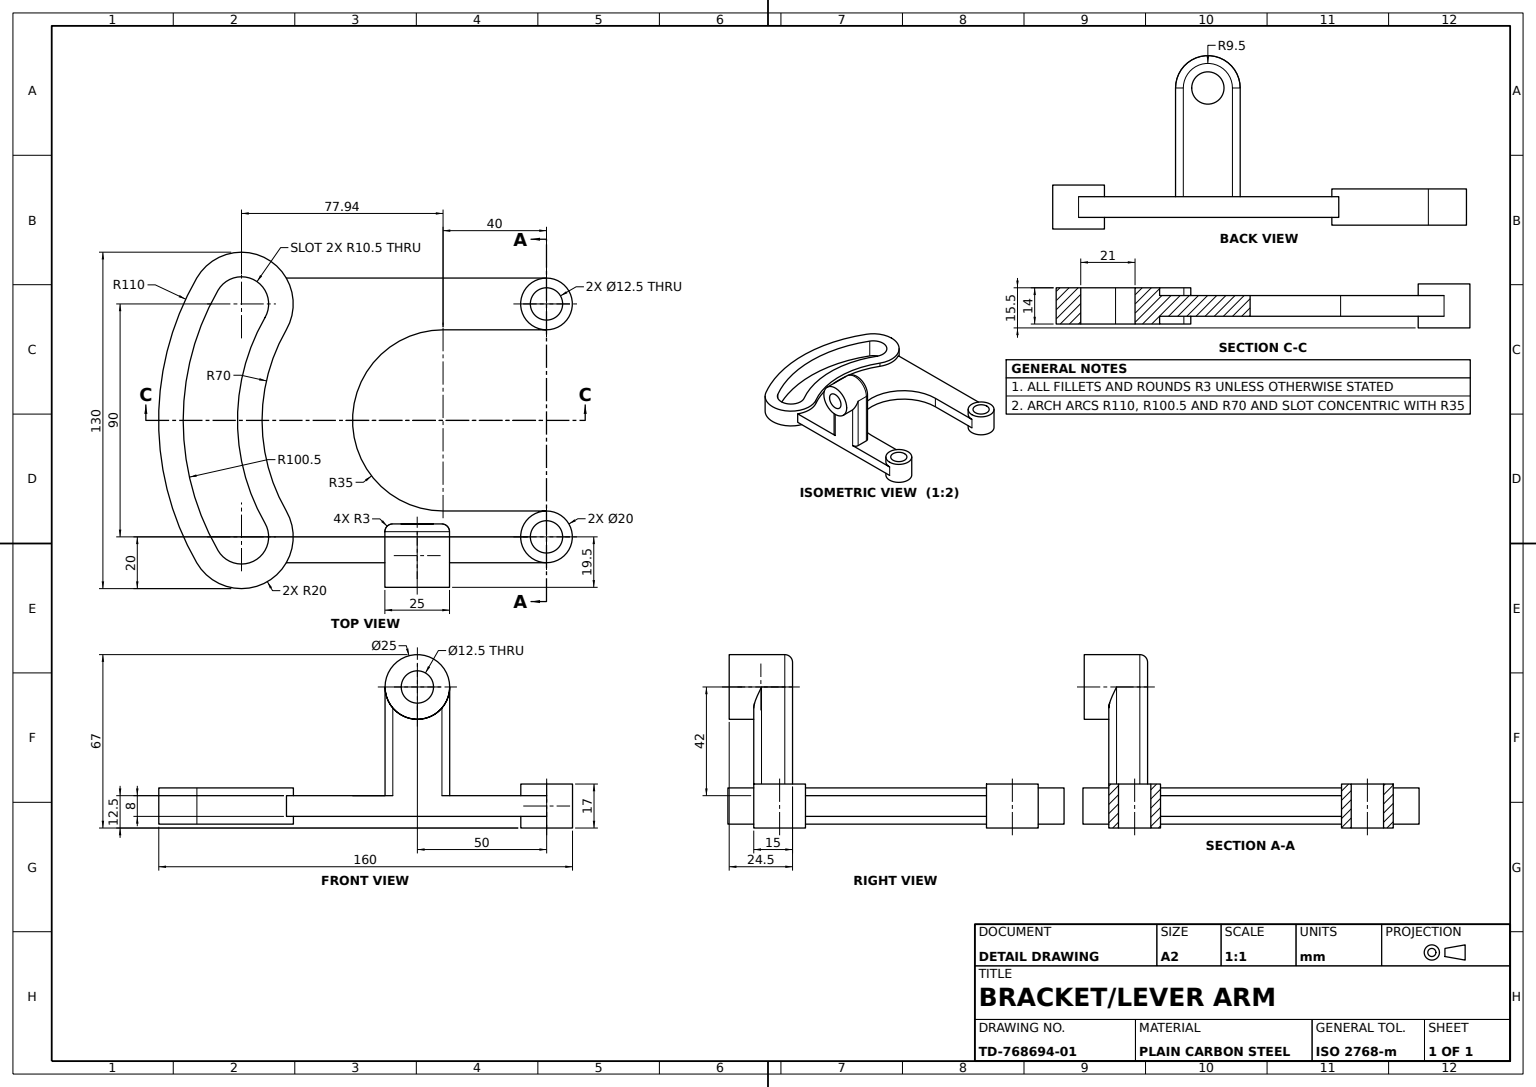
ISO-10303-21;
HEADER;
FILE_DESCRIPTION((''),'2;1');
FILE_NAME('','',(''),(''),'','','');
FILE_SCHEMA(('AUTOMOTIVE_DESIGN'));
ENDSEC;
DATA;
#1=APPLICATION_CONTEXT('');
#2=PRODUCT_CONTEXT('',#1,'mechanical');
#3=PRODUCT('','','',(#2));
#4=PRODUCT_DEFINITION_FORMATION('','',#3);
#5=PRODUCT_DEFINITION_CONTEXT('',#1,'design');
#6=PRODUCT_DEFINITION('','',#4,#5);
#7=PRODUCT_DEFINITION_SHAPE('','',#6);
#8=(LENGTH_UNIT()NAMED_UNIT(*)SI_UNIT(.MILLI.,.METRE.));
#9=(NAMED_UNIT(*)PLANE_ANGLE_UNIT()SI_UNIT($,.RADIAN.));
#10=(NAMED_UNIT(*)SI_UNIT($,.STERADIAN.)SOLID_ANGLE_UNIT());
#11=UNCERTAINTY_MEASURE_WITH_UNIT(LENGTH_MEASURE(1.E-05),#8,'distance_accuracy_value','');
#12=(GEOMETRIC_REPRESENTATION_CONTEXT(3)GLOBAL_UNCERTAINTY_ASSIGNED_CONTEXT((#11))GLOBAL_UNIT_ASSIGNED_CONTEXT((#8,#9,#10))REPRESENTATION_CONTEXT('',''));
#13=CARTESIAN_POINT('',(0.,-4.,-80.));
#14=VERTEX_POINT('',#13);
#15=CARTESIAN_POINT('',(0.,-8.5,-80.));
#16=VERTEX_POINT('',#15);
#17=CARTESIAN_POINT('',(0.,8.5,-80.));
#18=DIRECTION('',(0.,-1.,0.));
#19=VECTOR('',#18,1000.);
#20=LINE('',#17,#19);
#21=EDGE_CURVE('',#14,#16,#20,.T.);
#22=ORIENTED_EDGE('',*,*,#21,.T.);
#23=CARTESIAN_POINT('',(0.,-8.5,-100.));
#24=VERTEX_POINT('',#23);
#25=CARTESIAN_POINT('',(0.,-8.5,-90.));
#26=DIRECTION('',(0.,1.,0.));
#27=DIRECTION('',(0.,0.,1.));
#28=AXIS2_PLACEMENT_3D('',#25,#26,#27);
#29=CIRCLE('',#28,10.);
#30=EDGE_CURVE('',#16,#24,#29,.T.);
#31=ORIENTED_EDGE('',*,*,#30,.T.);
#32=CARTESIAN_POINT('',(0.,-4.,-100.));
#33=VERTEX_POINT('',#32);
#34=CARTESIAN_POINT('',(0.,8.5,-100.));
#35=LINE('',#34,#19);
#36=EDGE_CURVE('',#33,#24,#35,.T.);
#37=ORIENTED_EDGE('',*,*,#36,.F.);
#38=CARTESIAN_POINT('',(0.,4.,-100.));
#39=VERTEX_POINT('',#38);
#40=LINE('',#38,#19);
#41=EDGE_CURVE('',#39,#33,#40,.T.);
#42=ORIENTED_EDGE('',*,*,#41,.F.);
#43=VERTEX_POINT('',#34);
#44=EDGE_CURVE('',#43,#39,#35,.T.);
#45=ORIENTED_EDGE('',*,*,#44,.F.);
#46=VERTEX_POINT('',#17);
#47=CARTESIAN_POINT('',(0.,8.5,-90.));
#48=AXIS2_PLACEMENT_3D('',#47,#26,#27);
#49=CIRCLE('',#48,10.);
#50=EDGE_CURVE('',#46,#43,#49,.T.);
#51=ORIENTED_EDGE('',*,*,#50,.F.);
#52=CARTESIAN_POINT('',(0.,4.,-80.));
#53=VERTEX_POINT('',#52);
#54=EDGE_CURVE('',#46,#53,#20,.T.);
#55=ORIENTED_EDGE('',*,*,#54,.T.);
#56=LINE('',#52,#19);
#57=EDGE_CURVE('',#53,#14,#56,.T.);
#58=ORIENTED_EDGE('',*,*,#57,.T.);
#59=EDGE_LOOP('',(#22,#31,#37,#42,#45,#51,#55,#58));
#60=FACE_OUTER_BOUND('',#59,.T.);
#61=DIRECTION('',(0.,0.,-1.));
#62=AXIS2_PLACEMENT_3D('',#47,#18,#61);
#63=CYLINDRICAL_SURFACE('',#62,10.);
#64=ADVANCED_FACE('',(#60),#63,.T.);
#65=CARTESIAN_POINT('',(-117.942286,-7.,-110.));
#66=VERTEX_POINT('',#65);
#67=CARTESIAN_POINT('',(-135.262794,-7.,-100.));
#68=VERTEX_POINT('',#67);
#69=CARTESIAN_POINT('',(-117.942286,-7.,-90.));
#70=AXIS2_PLACEMENT_3D('',#69,#26,#27);
#71=CIRCLE('',#70,20.);
#72=EDGE_CURVE('',#66,#68,#71,.T.);
#73=ORIENTED_EDGE('',*,*,#72,.T.);
#74=CARTESIAN_POINT('',(-135.262794,7.,-100.));
#75=VERTEX_POINT('',#74);
#76=LINE('',#74,#19);
#77=EDGE_CURVE('',#75,#68,#76,.T.);
#78=ORIENTED_EDGE('',*,*,#77,.F.);
#79=CARTESIAN_POINT('',(-117.942286,7.,-110.));
#80=VERTEX_POINT('',#79);
#81=CARTESIAN_POINT('',(-117.942286,7.,-90.));
#82=AXIS2_PLACEMENT_3D('',#81,#26,#27);
#83=CIRCLE('',#82,20.);
#84=EDGE_CURVE('',#80,#75,#83,.T.);
#85=ORIENTED_EDGE('',*,*,#84,.F.);
#86=LINE('',#79,#19);
#87=EDGE_CURVE('',#80,#66,#86,.T.);
#88=ORIENTED_EDGE('',*,*,#87,.T.);
#89=EDGE_LOOP('',(#73,#78,#85,#88));
#90=FACE_OUTER_BOUND('',#89,.T.);
#91=AXIS2_PLACEMENT_3D('',#81,#18,#61);
#92=CYLINDRICAL_SURFACE('',#91,20.);
#93=ADVANCED_FACE('',(#90),#92,.T.);
#94=CARTESIAN_POINT('',(0.,-8.5,-96.25));
#95=VERTEX_POINT('',#94);
#96=CARTESIAN_POINT('',(0.,-8.5,-83.75));
#97=VERTEX_POINT('',#96);
#98=CIRCLE('',#28,6.25);
#99=EDGE_CURVE('',#95,#97,#98,.T.);
#100=ORIENTED_EDGE('',*,*,#99,.T.);
#101=EDGE_CURVE('',#97,#95,#98,.T.);
#102=ORIENTED_EDGE('',*,*,#101,.T.);
#103=EDGE_LOOP('',(#100,#102));
#104=FACE_BOUND('',#103,.T.);
#105=ORIENTED_EDGE('',*,*,#30,.F.);
#106=EDGE_CURVE('',#24,#16,#29,.T.);
#107=ORIENTED_EDGE('',*,*,#106,.F.);
#108=EDGE_LOOP('',(#105,#107));
#109=FACE_OUTER_BOUND('',#108,.T.);
#110=PLANE('',#28);
#111=ADVANCED_FACE('',(#104,#109),#110,.F.);
#112=CARTESIAN_POINT('',(-37.5,46.,19.5));
#113=VERTEX_POINT('',#112);
#114=CARTESIAN_POINT('',(-62.5,46.,19.5));
#115=VERTEX_POINT('',#114);
#116=CARTESIAN_POINT('',(-50.,46.,19.5));
#117=DIRECTION('',(1.,0.,0.));
#118=AXIS2_PLACEMENT_3D('',#116,#27,#117);
#119=CIRCLE('',#118,12.5);
#120=EDGE_CURVE('',#113,#115,#119,.T.);
#121=ORIENTED_EDGE('',*,*,#120,.T.);
#122=EDGE_CURVE('',#115,#113,#119,.T.);
#123=ORIENTED_EDGE('',*,*,#122,.T.);
#124=EDGE_LOOP('',(#121,#123));
#125=FACE_OUTER_BOUND('',#124,.T.);
#126=CARTESIAN_POINT('',(-56.25,46.,19.5));
#127=VERTEX_POINT('',#126);
#128=CARTESIAN_POINT('',(-43.75,46.,19.5));
#129=VERTEX_POINT('',#128);
#130=CIRCLE('',#118,6.25);
#131=EDGE_CURVE('',#127,#129,#130,.T.);
#132=ORIENTED_EDGE('',*,*,#131,.F.);
#133=EDGE_CURVE('',#129,#127,#130,.T.);
#134=ORIENTED_EDGE('',*,*,#133,.F.);
#135=EDGE_LOOP('',(#132,#134));
#136=FACE_BOUND('',#135,.T.);
#137=PLANE('',#118);
#138=ADVANCED_FACE('',(#125,#136),#137,.T.);
#139=CARTESIAN_POINT('',(-59.5,46.,-5.));
#140=VERTEX_POINT('',#139);
#141=CARTESIAN_POINT('',(-40.5,46.,-5.));
#142=VERTEX_POINT('',#141);
#143=CARTESIAN_POINT('',(-50.,46.,-5.));
#144=AXIS2_PLACEMENT_3D('',#143,#61,#117);
#145=CIRCLE('',#144,9.5);
#146=EDGE_CURVE('',#140,#142,#145,.T.);
#147=ORIENTED_EDGE('',*,*,#146,.F.);
#148=CARTESIAN_POINT('',(-62.5,46.,-2.));
#149=VERTEX_POINT('',#148);
#150=CARTESIAN_POINT('',(-59.5,46.,-2.));
#151=AXIS2_PLACEMENT_3D('',#150,#26,#27);
#152=CIRCLE('',#151,3.);
#153=EDGE_CURVE('',#140,#149,#152,.T.);
#154=ORIENTED_EDGE('',*,*,#153,.T.);
#155=CARTESIAN_POINT('',(-37.5,46.,-2.));
#156=VERTEX_POINT('',#155);
#157=CARTESIAN_POINT('',(-50.,46.,-2.));
#158=AXIS2_PLACEMENT_3D('',#157,#27,#117);
#159=CIRCLE('',#158,12.5);
#160=EDGE_CURVE('',#156,#149,#159,.T.);
#161=ORIENTED_EDGE('',*,*,#160,.F.);
#162=CARTESIAN_POINT('',(-40.5,46.,-2.));
#163=AXIS2_PLACEMENT_3D('',#162,#26,#27);
#164=CIRCLE('',#163,3.);
#165=EDGE_CURVE('',#156,#142,#164,.T.);
#166=ORIENTED_EDGE('',*,*,#165,.T.);
#167=EDGE_LOOP('',(#147,#154,#161,#166));
#168=FACE_OUTER_BOUND('',#167,.T.);
#169=TOROIDAL_SURFACE('',#158,9.5,3.);
#170=ADVANCED_FACE('',(#168),#169,.T.);
#171=ORIENTED_EDGE('',*,*,#54,.F.);
#172=EDGE_CURVE('',#43,#46,#49,.T.);
#173=ORIENTED_EDGE('',*,*,#172,.F.);
#174=ORIENTED_EDGE('',*,*,#44,.T.);
#175=CARTESIAN_POINT('',(0.,4.,-90.));
#176=AXIS2_PLACEMENT_3D('',#175,#18,#27);
#177=CIRCLE('',#176,10.);
#178=EDGE_CURVE('',#53,#39,#177,.T.);
#179=ORIENTED_EDGE('',*,*,#178,.F.);
#180=EDGE_LOOP('',(#171,#173,#174,#179));
#181=FACE_OUTER_BOUND('',#180,.T.);
#182=ADVANCED_FACE('',(#181),#63,.T.);
#183=CARTESIAN_POINT('',(-37.5,4.,7.));
#184=VERTEX_POINT('',#183);
#185=CARTESIAN_POINT('',(-37.5,4.,-2.));
#186=VERTEX_POINT('',#185);
#187=CARTESIAN_POINT('',(-37.5,4.,10.));
#188=VECTOR('',#61,1000.);
#189=LINE('',#187,#188);
#190=EDGE_CURVE('',#184,#186,#189,.T.);
#191=ORIENTED_EDGE('',*,*,#190,.T.);
#192=VECTOR('',#26,1000.);
#193=LINE('',#155,#192);
#194=EDGE_CURVE('',#186,#156,#193,.T.);
#195=ORIENTED_EDGE('',*,*,#194,.T.);
#196=CARTESIAN_POINT('',(-37.5,46.,7.));
#197=VERTEX_POINT('',#196);
#198=CARTESIAN_POINT('',(-37.5,46.,10.));
#199=LINE('',#198,#188);
#200=EDGE_CURVE('',#197,#156,#199,.T.);
#201=ORIENTED_EDGE('',*,*,#200,.F.);
#202=LINE('',#196,#19);
#203=EDGE_CURVE('',#197,#184,#202,.T.);
#204=ORIENTED_EDGE('',*,*,#203,.T.);
#205=EDGE_LOOP('',(#191,#195,#201,#204));
#206=FACE_OUTER_BOUND('',#205,.T.);
#207=DIRECTION('',(-1.,0.,0.));
#208=AXIS2_PLACEMENT_3D('',#198,#207,#27);
#209=PLANE('',#208);
#210=ADVANCED_FACE('',(#206),#209,.F.);
#211=CARTESIAN_POINT('',(0.,-8.5,-6.25));
#212=VERTEX_POINT('',#211);
#213=CARTESIAN_POINT('',(0.,-8.5,6.25));
#214=VERTEX_POINT('',#213);
#215=CARTESIAN_POINT('',(0.,-8.5,0.));
#216=AXIS2_PLACEMENT_3D('',#215,#26,#27);
#217=CIRCLE('',#216,6.25);
#218=EDGE_CURVE('',#212,#214,#217,.T.);
#219=ORIENTED_EDGE('',*,*,#218,.F.);
#220=CARTESIAN_POINT('',(0.,8.5,-6.25));
#221=VERTEX_POINT('',#220);
#222=LINE('',#220,#19);
#223=EDGE_CURVE('',#221,#212,#222,.T.);
#224=ORIENTED_EDGE('',*,*,#223,.F.);
#225=CARTESIAN_POINT('',(0.,8.5,6.25));
#226=VERTEX_POINT('',#225);
#227=CARTESIAN_POINT('',(0.,8.5,0.));
#228=AXIS2_PLACEMENT_3D('',#227,#26,#27);
#229=CIRCLE('',#228,6.25);
#230=EDGE_CURVE('',#221,#226,#229,.T.);
#231=ORIENTED_EDGE('',*,*,#230,.T.);
#232=LINE('',#225,#19);
#233=EDGE_CURVE('',#226,#214,#232,.T.);
#234=ORIENTED_EDGE('',*,*,#233,.T.);
#235=EDGE_LOOP('',(#219,#224,#231,#234));
#236=FACE_OUTER_BOUND('',#235,.T.);
#237=AXIS2_PLACEMENT_3D('',#227,#18,#61);
#238=CYLINDRICAL_SURFACE('',#237,6.25);
#239=ADVANCED_FACE('',(#236),#238,.F.);
#240=CARTESIAN_POINT('',(-56.25,46.,-5.));
#241=VERTEX_POINT('',#240);
#242=CARTESIAN_POINT('',(-56.25,46.,-40.355339));
#243=VECTOR('',#27,1000.);
#244=LINE('',#242,#243);
#245=EDGE_CURVE('',#241,#127,#244,.T.);
#246=ORIENTED_EDGE('',*,*,#245,.F.);
#247=CARTESIAN_POINT('',(-43.75,46.,-5.));
#248=VERTEX_POINT('',#247);
#249=CIRCLE('',#144,6.25);
#250=EDGE_CURVE('',#241,#248,#249,.T.);
#251=ORIENTED_EDGE('',*,*,#250,.T.);
#252=CARTESIAN_POINT('',(-43.75,46.,-40.355339));
#253=LINE('',#252,#243);
#254=EDGE_CURVE('',#248,#129,#253,.T.);
#255=ORIENTED_EDGE('',*,*,#254,.T.);
#256=ORIENTED_EDGE('',*,*,#133,.T.);
#257=EDGE_LOOP('',(#246,#251,#255,#256));
#258=FACE_OUTER_BOUND('',#257,.T.);
#259=CARTESIAN_POINT('',(-50.,46.,-40.355339));
#260=AXIS2_PLACEMENT_3D('',#259,#27,#117);
#261=CYLINDRICAL_SURFACE('',#260,6.25);
#262=ADVANCED_FACE('',(#258),#261,.F.);
#263=CARTESIAN_POINT('',(-100.621778,-4.,10.));
#264=VERTEX_POINT('',#263);
#265=CARTESIAN_POINT('',(-100.621778,4.,10.));
#266=VERTEX_POINT('',#265);
#267=CARTESIAN_POINT('',(-100.621778,7.,10.));
#268=LINE('',#267,#192);
#269=EDGE_CURVE('',#264,#266,#268,.T.);
#270=ORIENTED_EDGE('',*,*,#269,.T.);
#271=CARTESIAN_POINT('',(-100.621778,4.,-10.));
#272=VERTEX_POINT('',#271);
#273=CARTESIAN_POINT('',(-117.942286,4.,0.));
#274=AXIS2_PLACEMENT_3D('',#273,#18,#27);
#275=CIRCLE('',#274,20.);
#276=EDGE_CURVE('',#272,#266,#275,.T.);
#277=ORIENTED_EDGE('',*,*,#276,.F.);
#278=CARTESIAN_POINT('',(-100.621778,7.,-10.));
#279=VERTEX_POINT('',#278);
#280=LINE('',#278,#19);
#281=EDGE_CURVE('',#279,#272,#280,.T.);
#282=ORIENTED_EDGE('',*,*,#281,.F.);
#283=CARTESIAN_POINT('',(-135.262794,7.,10.));
#284=VERTEX_POINT('',#283);
#285=CARTESIAN_POINT('',(-117.942286,7.,0.));
#286=AXIS2_PLACEMENT_3D('',#285,#26,#27);
#287=CIRCLE('',#286,20.);
#288=EDGE_CURVE('',#284,#279,#287,.T.);
#289=ORIENTED_EDGE('',*,*,#288,.F.);
#290=CARTESIAN_POINT('',(-135.262794,-7.,10.));
#291=VERTEX_POINT('',#290);
#292=LINE('',#283,#19);
#293=EDGE_CURVE('',#284,#291,#292,.T.);
#294=ORIENTED_EDGE('',*,*,#293,.T.);
#295=CARTESIAN_POINT('',(-100.621778,-7.,-10.));
#296=VERTEX_POINT('',#295);
#297=CARTESIAN_POINT('',(-117.942286,-7.,0.));
#298=AXIS2_PLACEMENT_3D('',#297,#26,#27);
#299=CIRCLE('',#298,20.);
#300=EDGE_CURVE('',#291,#296,#299,.T.);
#301=ORIENTED_EDGE('',*,*,#300,.T.);
#302=CARTESIAN_POINT('',(-100.621778,-4.,-10.));
#303=VERTEX_POINT('',#302);
#304=EDGE_CURVE('',#303,#296,#280,.T.);
#305=ORIENTED_EDGE('',*,*,#304,.F.);
#306=CARTESIAN_POINT('',(-117.942286,-4.,0.));
#307=AXIS2_PLACEMENT_3D('',#306,#18,#27);
#308=CIRCLE('',#307,20.);
#309=EDGE_CURVE('',#303,#264,#308,.T.);
#310=ORIENTED_EDGE('',*,*,#309,.T.);
#311=EDGE_LOOP('',(#270,#277,#282,#289,#294,#301,#305,#310));
#312=FACE_OUTER_BOUND('',#311,.T.);
#313=AXIS2_PLACEMENT_3D('',#285,#18,#61);
#314=CYLINDRICAL_SURFACE('',#313,20.);
#315=ADVANCED_FACE('',(#312),#314,.T.);
#316=ORIENTED_EDGE('',*,*,#41,.T.);
#317=CARTESIAN_POINT('',(-100.621778,-4.,-100.));
#318=VERTEX_POINT('',#317);
#319=VECTOR('',#207,1000.);
#320=LINE('',#32,#319);
#321=EDGE_CURVE('',#33,#318,#320,.T.);
#322=ORIENTED_EDGE('',*,*,#321,.T.);
#323=CARTESIAN_POINT('',(-100.621778,4.,-100.));
#324=VERTEX_POINT('',#323);
#325=CARTESIAN_POINT('',(-100.621778,7.,-100.));
#326=LINE('',#325,#19);
#327=EDGE_CURVE('',#324,#318,#326,.T.);
#328=ORIENTED_EDGE('',*,*,#327,.F.);
#329=LINE('',#38,#319);
#330=EDGE_CURVE('',#39,#324,#329,.T.);
#331=ORIENTED_EDGE('',*,*,#330,.F.);
#332=EDGE_LOOP('',(#316,#322,#328,#331));
#333=FACE_OUTER_BOUND('',#332,.T.);
#334=AXIS2_PLACEMENT_3D('',#38,#27,#117);
#335=PLANE('',#334);
#336=ADVANCED_FACE('',(#333),#335,.F.);
#337=CARTESIAN_POINT('',(-108.84902,7.,-5.25));
#338=VERTEX_POINT('',#337);
#339=CARTESIAN_POINT('',(-108.84902,7.,-84.75));
#340=VERTEX_POINT('',#339);
#341=CARTESIAN_POINT('',(-40.,7.,-45.));
#342=AXIS2_PLACEMENT_3D('',#341,#18,#27);
#343=CIRCLE('',#342,79.5);
#344=EDGE_CURVE('',#338,#340,#343,.T.);
#345=ORIENTED_EDGE('',*,*,#344,.T.);
#346=CARTESIAN_POINT('',(-108.84902,-7.,-84.75));
#347=VERTEX_POINT('',#346);
#348=LINE('',#339,#19);
#349=EDGE_CURVE('',#340,#347,#348,.T.);
#350=ORIENTED_EDGE('',*,*,#349,.T.);
#351=CARTESIAN_POINT('',(-108.84902,-7.,-5.25));
#352=VERTEX_POINT('',#351);
#353=CARTESIAN_POINT('',(-40.,-7.,-45.));
#354=AXIS2_PLACEMENT_3D('',#353,#18,#27);
#355=CIRCLE('',#354,79.5);
#356=EDGE_CURVE('',#352,#347,#355,.T.);
#357=ORIENTED_EDGE('',*,*,#356,.F.);
#358=LINE('',#337,#19);
#359=EDGE_CURVE('',#338,#352,#358,.T.);
#360=ORIENTED_EDGE('',*,*,#359,.F.);
#361=EDGE_LOOP('',(#345,#350,#357,#360));
#362=FACE_OUTER_BOUND('',#361,.T.);
#363=AXIS2_PLACEMENT_3D('',#341,#18,#61);
#364=CYLINDRICAL_SURFACE('',#363,79.5);
#365=ADVANCED_FACE('',(#362),#364,.T.);
#366=CARTESIAN_POINT('',(-127.035553,7.,5.25));
#367=VERTEX_POINT('',#366);
#368=CARTESIAN_POINT('',(-127.035553,-7.,5.25));
#369=VERTEX_POINT('',#368);
#370=LINE('',#366,#19);
#371=EDGE_CURVE('',#367,#369,#370,.T.);
#372=ORIENTED_EDGE('',*,*,#371,.T.);
#373=CARTESIAN_POINT('',(-127.035553,-7.,-95.25));
#374=VERTEX_POINT('',#373);
#375=AXIS2_PLACEMENT_3D('',#353,#26,#27);
#376=CIRCLE('',#375,100.5);
#377=EDGE_CURVE('',#374,#369,#376,.T.);
#378=ORIENTED_EDGE('',*,*,#377,.F.);
#379=CARTESIAN_POINT('',(-127.035553,7.,-95.25));
#380=VERTEX_POINT('',#379);
#381=LINE('',#379,#19);
#382=EDGE_CURVE('',#380,#374,#381,.T.);
#383=ORIENTED_EDGE('',*,*,#382,.F.);
#384=AXIS2_PLACEMENT_3D('',#341,#26,#27);
#385=CIRCLE('',#384,100.5);
#386=EDGE_CURVE('',#380,#367,#385,.T.);
#387=ORIENTED_EDGE('',*,*,#386,.T.);
#388=EDGE_LOOP('',(#372,#378,#383,#387));
#389=FACE_OUTER_BOUND('',#388,.T.);
#390=CYLINDRICAL_SURFACE('',#363,100.5);
#391=ADVANCED_FACE('',(#389),#390,.F.);
#392=ORIENTED_EDGE('',*,*,#218,.T.);
#393=EDGE_CURVE('',#214,#212,#217,.T.);
#394=ORIENTED_EDGE('',*,*,#393,.T.);
#395=EDGE_LOOP('',(#392,#394));
#396=FACE_BOUND('',#395,.T.);
#397=CARTESIAN_POINT('',(0.,-8.5,10.));
#398=VERTEX_POINT('',#397);
#399=CARTESIAN_POINT('',(0.,-8.5,-10.));
#400=VERTEX_POINT('',#399);
#401=CIRCLE('',#216,10.);
#402=EDGE_CURVE('',#398,#400,#401,.T.);
#403=ORIENTED_EDGE('',*,*,#402,.F.);
#404=EDGE_CURVE('',#400,#398,#401,.T.);
#405=ORIENTED_EDGE('',*,*,#404,.F.);
#406=EDGE_LOOP('',(#403,#405));
#407=FACE_OUTER_BOUND('',#406,.T.);
#408=PLANE('',#216);
#409=ADVANCED_FACE('',(#396,#407),#408,.F.);
#410=CARTESIAN_POINT('',(-100.621778,7.,-80.));
#411=VERTEX_POINT('',#410);
#412=EDGE_CURVE('',#411,#80,#83,.T.);
#413=ORIENTED_EDGE('',*,*,#412,.T.);
#414=ORIENTED_EDGE('',*,*,#84,.T.);
#415=CIRCLE('',#384,110.);
#416=EDGE_CURVE('',#75,#284,#415,.T.);
#417=ORIENTED_EDGE('',*,*,#416,.T.);
#418=ORIENTED_EDGE('',*,*,#288,.T.);
#419=CIRCLE('',#342,70.);
#420=EDGE_CURVE('',#279,#411,#419,.T.);
#421=ORIENTED_EDGE('',*,*,#420,.T.);
#422=EDGE_LOOP('',(#413,#414,#417,#418,#421));
#423=FACE_OUTER_BOUND('',#422,.T.);
#424=CARTESIAN_POINT('',(-117.942286,7.,-100.5));
#425=VERTEX_POINT('',#424);
#426=CIRCLE('',#82,10.5);
#427=EDGE_CURVE('',#425,#380,#426,.T.);
#428=ORIENTED_EDGE('',*,*,#427,.F.);
#429=EDGE_CURVE('',#340,#425,#426,.T.);
#430=ORIENTED_EDGE('',*,*,#429,.F.);
#431=ORIENTED_EDGE('',*,*,#344,.F.);
#432=CIRCLE('',#286,10.5);
#433=EDGE_CURVE('',#367,#338,#432,.T.);
#434=ORIENTED_EDGE('',*,*,#433,.F.);
#435=ORIENTED_EDGE('',*,*,#386,.F.);
#436=EDGE_LOOP('',(#428,#430,#431,#434,#435));
#437=FACE_BOUND('',#436,.T.);
#438=CARTESIAN_POINT('',(-78.971143,7.,-67.5));
#439=AXIS2_PLACEMENT_3D('',#438,#26,#27);
#440=PLANE('',#439);
#441=ADVANCED_FACE('',(#423,#437),#440,.T.);
#442=CIRCLE('',#298,10.5);
#443=EDGE_CURVE('',#369,#352,#442,.T.);
#444=ORIENTED_EDGE('',*,*,#443,.F.);
#445=ORIENTED_EDGE('',*,*,#371,.F.);
#446=ORIENTED_EDGE('',*,*,#433,.T.);
#447=ORIENTED_EDGE('',*,*,#359,.T.);
#448=EDGE_LOOP('',(#444,#445,#446,#447));
#449=FACE_OUTER_BOUND('',#448,.T.);
#450=CYLINDRICAL_SURFACE('',#313,10.5);
#451=ADVANCED_FACE('',(#449),#450,.F.);
#452=CARTESIAN_POINT('',(0.,-4.,10.));
#453=VERTEX_POINT('',#452);
#454=VECTOR('',#117,1000.);
#455=LINE('',#452,#454);
#456=EDGE_CURVE('',#264,#453,#455,.T.);
#457=ORIENTED_EDGE('',*,*,#456,.F.);
#458=ORIENTED_EDGE('',*,*,#309,.F.);
#459=CARTESIAN_POINT('',(-100.621778,-4.,-80.));
#460=VERTEX_POINT('',#459);
#461=CARTESIAN_POINT('',(-40.,-4.,-45.));
#462=AXIS2_PLACEMENT_3D('',#461,#26,#27);
#463=CIRCLE('',#462,70.);
#464=EDGE_CURVE('',#460,#303,#463,.T.);
#465=ORIENTED_EDGE('',*,*,#464,.F.);
#466=CARTESIAN_POINT('',(-117.942286,-4.,-90.));
#467=AXIS2_PLACEMENT_3D('',#466,#18,#27);
#468=CIRCLE('',#467,20.);
#469=EDGE_CURVE('',#318,#460,#468,.T.);
#470=ORIENTED_EDGE('',*,*,#469,.F.);
#471=ORIENTED_EDGE('',*,*,#321,.F.);
#472=CARTESIAN_POINT('',(0.,-4.,-90.));
#473=AXIS2_PLACEMENT_3D('',#472,#18,#27);
#474=CIRCLE('',#473,10.);
#475=EDGE_CURVE('',#14,#33,#474,.T.);
#476=ORIENTED_EDGE('',*,*,#475,.F.);
#477=CARTESIAN_POINT('',(-40.,-4.,-80.));
#478=VERTEX_POINT('',#477);
#479=LINE('',#13,#454);
#480=EDGE_CURVE('',#478,#14,#479,.T.);
#481=ORIENTED_EDGE('',*,*,#480,.F.);
#482=CARTESIAN_POINT('',(-40.,-4.,-10.));
#483=VERTEX_POINT('',#482);
#484=AXIS2_PLACEMENT_3D('',#461,#18,#27);
#485=CIRCLE('',#484,35.);
#486=EDGE_CURVE('',#483,#478,#485,.T.);
#487=ORIENTED_EDGE('',*,*,#486,.F.);
#488=CARTESIAN_POINT('',(0.,-4.,-10.));
#489=VERTEX_POINT('',#488);
#490=LINE('',#482,#319);
#491=EDGE_CURVE('',#489,#483,#490,.T.);
#492=ORIENTED_EDGE('',*,*,#491,.F.);
#493=CARTESIAN_POINT('',(0.,-4.,0.));
#494=AXIS2_PLACEMENT_3D('',#493,#18,#27);
#495=CIRCLE('',#494,10.);
#496=EDGE_CURVE('',#453,#489,#495,.T.);
#497=ORIENTED_EDGE('',*,*,#496,.F.);
#498=EDGE_LOOP('',(#457,#458,#465,#470,#471,#476,#481,#487,#492,#497));
#499=FACE_OUTER_BOUND('',#498,.T.);
#500=AXIS2_PLACEMENT_3D('',#472,#26,#27);
#501=PLANE('',#500);
#502=ADVANCED_FACE('',(#499),#501,.F.);
#503=CARTESIAN_POINT('',(-40.5,4.,10.));
#504=VERTEX_POINT('',#503);
#505=CARTESIAN_POINT('',(0.,4.,10.));
#506=VERTEX_POINT('',#505);
#507=LINE('',#505,#454);
#508=EDGE_CURVE('',#504,#506,#507,.T.);
#509=ORIENTED_EDGE('',*,*,#508,.F.);
#510=CARTESIAN_POINT('',(-40.5,37.875962,10.));
#511=VERTEX_POINT('',#510);
#512=LINE('',#503,#192);
#513=EDGE_CURVE('',#504,#511,#512,.T.);
#514=ORIENTED_EDGE('',*,*,#513,.T.);
#515=CARTESIAN_POINT('',(-59.5,37.875962,10.));
#516=VERTEX_POINT('',#515);
#517=CARTESIAN_POINT('',(-50.,46.,10.));
#518=AXIS2_PLACEMENT_3D('',#517,#61,#207);
#519=CIRCLE('',#518,12.5);
#520=EDGE_CURVE('',#511,#516,#519,.T.);
#521=ORIENTED_EDGE('',*,*,#520,.T.);
#522=CARTESIAN_POINT('',(-59.5,4.,10.));
#523=VERTEX_POINT('',#522);
#524=LINE('',#522,#19);
#525=EDGE_CURVE('',#516,#523,#524,.T.);
#526=ORIENTED_EDGE('',*,*,#525,.T.);
#527=EDGE_CURVE('',#266,#523,#507,.T.);
#528=ORIENTED_EDGE('',*,*,#527,.F.);
#529=ORIENTED_EDGE('',*,*,#269,.F.);
#530=ORIENTED_EDGE('',*,*,#456,.T.);
#531=LINE('',#505,#19);
#532=EDGE_CURVE('',#506,#453,#531,.T.);
#533=ORIENTED_EDGE('',*,*,#532,.F.);
#534=EDGE_LOOP('',(#509,#514,#521,#526,#528,#529,#530,#533));
#535=FACE_OUTER_BOUND('',#534,.T.);
#536=AXIS2_PLACEMENT_3D('',#505,#61,#207);
#537=PLANE('',#536);
#538=ADVANCED_FACE('',(#535),#537,.F.);
#539=ORIENTED_EDGE('',*,*,#160,.T.);
#540=CARTESIAN_POINT('',(-62.5,46.,7.));
#541=VERTEX_POINT('',#540);
#542=CARTESIAN_POINT('',(-62.5,46.,10.));
#543=LINE('',#542,#243);
#544=EDGE_CURVE('',#149,#541,#543,.T.);
#545=ORIENTED_EDGE('',*,*,#544,.T.);
#546=CARTESIAN_POINT('',(-62.5,46.,-40.355339));
#547=LINE('',#546,#243);
#548=EDGE_CURVE('',#541,#115,#547,.T.);
#549=ORIENTED_EDGE('',*,*,#548,.T.);
#550=ORIENTED_EDGE('',*,*,#120,.F.);
#551=CARTESIAN_POINT('',(-37.5,46.,-40.355339));
#552=LINE('',#551,#243);
#553=EDGE_CURVE('',#197,#113,#552,.T.);
#554=ORIENTED_EDGE('',*,*,#553,.F.);
#555=ORIENTED_EDGE('',*,*,#200,.T.);
#556=EDGE_LOOP('',(#539,#545,#549,#550,#554,#555));
#557=FACE_OUTER_BOUND('',#556,.T.);
#558=CYLINDRICAL_SURFACE('',#260,12.5);
#559=ADVANCED_FACE('',(#557),#558,.T.);
#560=CARTESIAN_POINT('',(-100.621778,4.,-80.));
#561=VERTEX_POINT('',#560);
#562=LINE('',#410,#19);
#563=EDGE_CURVE('',#411,#561,#562,.T.);
#564=ORIENTED_EDGE('',*,*,#563,.F.);
#565=ORIENTED_EDGE('',*,*,#420,.F.);
#566=ORIENTED_EDGE('',*,*,#281,.T.);
#567=CARTESIAN_POINT('',(-40.,4.,-45.));
#568=AXIS2_PLACEMENT_3D('',#567,#26,#27);
#569=CIRCLE('',#568,70.);
#570=EDGE_CURVE('',#561,#272,#569,.T.);
#571=ORIENTED_EDGE('',*,*,#570,.F.);
#572=EDGE_LOOP('',(#564,#565,#566,#571));
#573=FACE_OUTER_BOUND('',#572,.T.);
#574=CYLINDRICAL_SURFACE('',#363,70.);
#575=ADVANCED_FACE('',(#573),#574,.F.);
#576=CARTESIAN_POINT('',(0.,4.,-10.));
#577=VERTEX_POINT('',#576);
#578=LINE('',#576,#19);
#579=EDGE_CURVE('',#577,#489,#578,.T.);
#580=ORIENTED_EDGE('',*,*,#579,.F.);
#581=CARTESIAN_POINT('',(0.,8.5,-10.));
#582=VERTEX_POINT('',#581);
#583=LINE('',#581,#19);
#584=EDGE_CURVE('',#582,#577,#583,.T.);
#585=ORIENTED_EDGE('',*,*,#584,.F.);
#586=CARTESIAN_POINT('',(0.,8.5,10.));
#587=VERTEX_POINT('',#586);
#588=CIRCLE('',#228,10.);
#589=EDGE_CURVE('',#587,#582,#588,.T.);
#590=ORIENTED_EDGE('',*,*,#589,.F.);
#591=LINE('',#586,#19);
#592=EDGE_CURVE('',#587,#506,#591,.T.);
#593=ORIENTED_EDGE('',*,*,#592,.T.);
#594=ORIENTED_EDGE('',*,*,#532,.T.);
#595=EDGE_CURVE('',#453,#398,#591,.T.);
#596=ORIENTED_EDGE('',*,*,#595,.T.);
#597=ORIENTED_EDGE('',*,*,#402,.T.);
#598=EDGE_CURVE('',#489,#400,#583,.T.);
#599=ORIENTED_EDGE('',*,*,#598,.F.);
#600=EDGE_LOOP('',(#580,#585,#590,#593,#594,#596,#597,#599));
#601=FACE_OUTER_BOUND('',#600,.T.);
#602=CYLINDRICAL_SURFACE('',#237,10.);
#603=ADVANCED_FACE('',(#601),#602,.T.);
#604=CARTESIAN_POINT('',(0.,8.5,-83.75));
#605=VERTEX_POINT('',#604);
#606=CARTESIAN_POINT('',(0.,8.5,-96.25));
#607=VERTEX_POINT('',#606);
#608=CIRCLE('',#48,6.25);
#609=EDGE_CURVE('',#605,#607,#608,.T.);
#610=ORIENTED_EDGE('',*,*,#609,.T.);
#611=LINE('',#606,#19);
#612=EDGE_CURVE('',#607,#95,#611,.T.);
#613=ORIENTED_EDGE('',*,*,#612,.T.);
#614=ORIENTED_EDGE('',*,*,#101,.F.);
#615=LINE('',#604,#19);
#616=EDGE_CURVE('',#605,#97,#615,.T.);
#617=ORIENTED_EDGE('',*,*,#616,.F.);
#618=EDGE_LOOP('',(#610,#613,#614,#617));
#619=FACE_OUTER_BOUND('',#618,.T.);
#620=CYLINDRICAL_SURFACE('',#62,6.25);
#621=ADVANCED_FACE('',(#619),#620,.F.);
#622=ORIENTED_EDGE('',*,*,#377,.T.);
#623=ORIENTED_EDGE('',*,*,#443,.T.);
#624=ORIENTED_EDGE('',*,*,#356,.T.);
#625=CARTESIAN_POINT('',(-117.942286,-7.,-100.5));
#626=VERTEX_POINT('',#625);
#627=CIRCLE('',#70,10.5);
#628=EDGE_CURVE('',#347,#626,#627,.T.);
#629=ORIENTED_EDGE('',*,*,#628,.T.);
#630=EDGE_CURVE('',#626,#374,#627,.T.);
#631=ORIENTED_EDGE('',*,*,#630,.T.);
#632=EDGE_LOOP('',(#622,#623,#624,#629,#631));
#633=FACE_BOUND('',#632,.T.);
#634=CARTESIAN_POINT('',(-100.621778,-7.,-80.));
#635=VERTEX_POINT('',#634);
#636=EDGE_CURVE('',#635,#66,#71,.T.);
#637=ORIENTED_EDGE('',*,*,#636,.F.);
#638=CIRCLE('',#354,70.);
#639=EDGE_CURVE('',#296,#635,#638,.T.);
#640=ORIENTED_EDGE('',*,*,#639,.F.);
#641=ORIENTED_EDGE('',*,*,#300,.F.);
#642=CIRCLE('',#375,110.);
#643=EDGE_CURVE('',#68,#291,#642,.T.);
#644=ORIENTED_EDGE('',*,*,#643,.F.);
#645=ORIENTED_EDGE('',*,*,#72,.F.);
#646=EDGE_LOOP('',(#637,#640,#641,#644,#645));
#647=FACE_OUTER_BOUND('',#646,.T.);
#648=CARTESIAN_POINT('',(-78.971143,-7.,-67.5));
#649=AXIS2_PLACEMENT_3D('',#648,#26,#27);
#650=PLANE('',#649);
#651=ADVANCED_FACE('',(#633,#647),#650,.F.);
#652=ORIENTED_EDGE('',*,*,#36,.T.);
#653=ORIENTED_EDGE('',*,*,#106,.T.);
#654=ORIENTED_EDGE('',*,*,#21,.F.);
#655=ORIENTED_EDGE('',*,*,#475,.T.);
#656=EDGE_LOOP('',(#652,#653,#654,#655));
#657=FACE_OUTER_BOUND('',#656,.T.);
#658=ADVANCED_FACE('',(#657),#63,.T.);
#659=CARTESIAN_POINT('',(-62.5,45.648021,7.172434));
#660=CARTESIAN_POINT('',(-62.485015,45.293609,7.34606));
#661=CARTESIAN_POINT('',(-62.425261,44.590221,7.687692));
#662=CARTESIAN_POINT('',(-62.380497,44.239376,7.856627));
#663=CARTESIAN_POINT('',(-62.260348,43.538215,8.188089));
#664=CARTESIAN_POINT('',(-62.184626,43.186682,8.351175));
#665=CARTESIAN_POINT('',(-62.002305,42.489366,8.664741));
#666=CARTESIAN_POINT('',(-61.89598,42.144126,8.815021));
#667=CARTESIAN_POINT('',(-61.529765,41.117076,9.240568));
#668=CARTESIAN_POINT('',(-61.223106,40.442997,9.492614));
#669=CARTESIAN_POINT('',(-60.650355,39.445076,9.778891));
#670=CARTESIAN_POINT('',(-60.443777,39.120488,9.85694));
#671=CARTESIAN_POINT('',(-59.99758,38.486774,9.967362));
#672=CARTESIAN_POINT('',(-59.758004,38.177663,10.));
#673=B_SPLINE_CURVE_WITH_KNOTS('',3,(#540,#659,#660,#661,#662,#663,#664,#665,#666,#667,#668,#669,#670,#671,#672,#515),.UNSPECIFIED.,.F.,.F.,(4,2,2,2,2,2,2,4),(-0.000022361,0.001153481,0.002329323,0.003505164,0.004681006,0.00703269,0.008208531,0.009384373),.UNSPECIFIED.);
#674=EDGE_CURVE('',#541,#516,#673,.T.);
#675=ORIENTED_EDGE('',*,*,#674,.F.);
#676=CARTESIAN_POINT('',(-62.5,4.,7.));
#677=VERTEX_POINT('',#676);
#678=LINE('',#540,#192);
#679=EDGE_CURVE('',#677,#541,#678,.T.);
#680=ORIENTED_EDGE('',*,*,#679,.F.);
#681=CARTESIAN_POINT('',(-59.5,4.,7.));
#682=AXIS2_PLACEMENT_3D('',#681,#18,#27);
#683=CIRCLE('',#682,3.);
#684=EDGE_CURVE('',#523,#677,#683,.T.);
#685=ORIENTED_EDGE('',*,*,#684,.F.);
#686=ORIENTED_EDGE('',*,*,#525,.F.);
#687=EDGE_LOOP('',(#675,#680,#685,#686));
#688=FACE_OUTER_BOUND('',#687,.T.);
#689=AXIS2_PLACEMENT_3D('',#681,#18,#61);
#690=CYLINDRICAL_SURFACE('',#689,3.);
#691=ADVANCED_FACE('',(#688),#690,.T.);
#692=CARTESIAN_POINT('',(-40.,4.,-80.));
#693=VERTEX_POINT('',#692);
#694=LINE('',#692,#19);
#695=EDGE_CURVE('',#693,#478,#694,.T.);
#696=ORIENTED_EDGE('',*,*,#695,.F.);
#697=CARTESIAN_POINT('',(-40.,4.,-10.));
#698=VERTEX_POINT('',#697);
#699=AXIS2_PLACEMENT_3D('',#567,#18,#27);
#700=CIRCLE('',#699,35.);
#701=EDGE_CURVE('',#698,#693,#700,.T.);
#702=ORIENTED_EDGE('',*,*,#701,.F.);
#703=LINE('',#697,#19);
#704=EDGE_CURVE('',#698,#483,#703,.T.);
#705=ORIENTED_EDGE('',*,*,#704,.T.);
#706=ORIENTED_EDGE('',*,*,#486,.T.);
#707=EDGE_LOOP('',(#696,#702,#705,#706));
#708=FACE_OUTER_BOUND('',#707,.T.);
#709=AXIS2_PLACEMENT_3D('',#567,#18,#61);
#710=CYLINDRICAL_SURFACE('',#709,35.);
#711=ADVANCED_FACE('',(#708),#710,.F.);
#712=ORIENTED_EDGE('',*,*,#233,.F.);
#713=EDGE_CURVE('',#226,#221,#229,.T.);
#714=ORIENTED_EDGE('',*,*,#713,.T.);
#715=ORIENTED_EDGE('',*,*,#223,.T.);
#716=ORIENTED_EDGE('',*,*,#393,.F.);
#717=EDGE_LOOP('',(#712,#714,#715,#716));
#718=FACE_OUTER_BOUND('',#717,.T.);
#719=ADVANCED_FACE('',(#718),#238,.F.);
#720=ORIENTED_EDGE('',*,*,#245,.T.);
#721=ORIENTED_EDGE('',*,*,#131,.T.);
#722=ORIENTED_EDGE('',*,*,#254,.F.);
#723=EDGE_CURVE('',#248,#241,#249,.T.);
#724=ORIENTED_EDGE('',*,*,#723,.T.);
#725=EDGE_LOOP('',(#720,#721,#722,#724));
#726=FACE_OUTER_BOUND('',#725,.T.);
#727=ADVANCED_FACE('',(#726),#261,.F.);
#728=LINE('',#424,#19);
#729=EDGE_CURVE('',#425,#626,#728,.T.);
#730=ORIENTED_EDGE('',*,*,#729,.T.);
#731=ORIENTED_EDGE('',*,*,#628,.F.);
#732=ORIENTED_EDGE('',*,*,#349,.F.);
#733=ORIENTED_EDGE('',*,*,#429,.T.);
#734=EDGE_LOOP('',(#730,#731,#732,#733));
#735=FACE_OUTER_BOUND('',#734,.T.);
#736=CYLINDRICAL_SURFACE('',#91,10.5);
#737=ADVANCED_FACE('',(#735),#736,.F.);
#738=CARTESIAN_POINT('',(-40.5,4.,7.));
#739=AXIS2_PLACEMENT_3D('',#738,#18,#27);
#740=CIRCLE('',#739,3.);
#741=EDGE_CURVE('',#184,#504,#740,.T.);
#742=ORIENTED_EDGE('',*,*,#741,.F.);
#743=ORIENTED_EDGE('',*,*,#203,.F.);
#744=CARTESIAN_POINT('',(-40.241996,38.177664,10.));
#745=CARTESIAN_POINT('',(-40.002418,38.486776,9.967361));
#746=CARTESIAN_POINT('',(-39.55622,39.120492,9.856939));
#747=CARTESIAN_POINT('',(-39.349641,39.445081,9.77889));
#748=CARTESIAN_POINT('',(-38.776889,40.443005,9.492612));
#749=CARTESIAN_POINT('',(-38.470231,41.117086,9.240564));
#750=CARTESIAN_POINT('',(-38.104015,42.14414,8.815015));
#751=CARTESIAN_POINT('',(-37.997691,42.489382,8.664734));
#752=CARTESIAN_POINT('',(-37.81537,43.1867,8.351167));
#753=CARTESIAN_POINT('',(-37.739648,43.538234,8.18808));
#754=CARTESIAN_POINT('',(-37.619499,44.239397,7.856617));
#755=CARTESIAN_POINT('',(-37.574737,44.590243,7.687681));
#756=CARTESIAN_POINT('',(-37.529922,45.117786,7.431457));
#757=CARTESIAN_POINT('',(-37.518714,45.293845,7.345574));
#758=CARTESIAN_POINT('',(-37.503752,45.64653,7.173164));
#759=CARTESIAN_POINT('',(-37.5,45.824242,7.086103));
#760=B_SPLINE_CURVE_WITH_KNOTS('',3,(#510,#744,#745,#746,#747,#748,#749,#750,#751,#752,#753,#754,#755,#756,#757,#758,#759,#196),.UNSPECIFIED.,.F.,.F.,(4,2,2,2,2,2,2,2,4),(0.,0.001174292,0.002348585,0.00469717,0.005871462,0.007045754,0.008220047,0.008807193,0.009394339),.UNSPECIFIED.);
#761=EDGE_CURVE('',#511,#197,#760,.T.);
#762=ORIENTED_EDGE('',*,*,#761,.F.);
#763=ORIENTED_EDGE('',*,*,#513,.F.);
#764=EDGE_LOOP('',(#742,#743,#762,#763));
#765=FACE_OUTER_BOUND('',#764,.T.);
#766=CARTESIAN_POINT('',(-40.5,46.,7.));
#767=AXIS2_PLACEMENT_3D('',#766,#18,#61);
#768=CYLINDRICAL_SURFACE('',#767,3.);
#769=ADVANCED_FACE('',(#765),#768,.T.);
#770=ORIENTED_EDGE('',*,*,#548,.F.);
#771=ORIENTED_EDGE('',*,*,#674,.T.);
#772=ORIENTED_EDGE('',*,*,#520,.F.);
#773=ORIENTED_EDGE('',*,*,#761,.T.);
#774=ORIENTED_EDGE('',*,*,#553,.T.);
#775=ORIENTED_EDGE('',*,*,#122,.F.);
#776=EDGE_LOOP('',(#770,#771,#772,#773,#774,#775));
#777=FACE_OUTER_BOUND('',#776,.T.);
#778=ADVANCED_FACE('',(#777),#558,.T.);
#779=ORIENTED_EDGE('',*,*,#404,.T.);
#780=ORIENTED_EDGE('',*,*,#595,.F.);
#781=ORIENTED_EDGE('',*,*,#496,.T.);
#782=ORIENTED_EDGE('',*,*,#598,.T.);
#783=EDGE_LOOP('',(#779,#780,#781,#782));
#784=FACE_OUTER_BOUND('',#783,.T.);
#785=ADVANCED_FACE('',(#784),#602,.T.);
#786=LINE('',#697,#319);
#787=EDGE_CURVE('',#577,#698,#786,.T.);
#788=ORIENTED_EDGE('',*,*,#787,.T.);
#789=ORIENTED_EDGE('',*,*,#701,.T.);
#790=LINE('',#52,#454);
#791=EDGE_CURVE('',#693,#53,#790,.T.);
#792=ORIENTED_EDGE('',*,*,#791,.T.);
#793=ORIENTED_EDGE('',*,*,#178,.T.);
#794=ORIENTED_EDGE('',*,*,#330,.T.);
#795=CARTESIAN_POINT('',(-117.942286,4.,-90.));
#796=AXIS2_PLACEMENT_3D('',#795,#18,#27);
#797=CIRCLE('',#796,20.);
#798=EDGE_CURVE('',#324,#561,#797,.T.);
#799=ORIENTED_EDGE('',*,*,#798,.T.);
#800=ORIENTED_EDGE('',*,*,#570,.T.);
#801=ORIENTED_EDGE('',*,*,#276,.T.);
#802=ORIENTED_EDGE('',*,*,#527,.T.);
#803=ORIENTED_EDGE('',*,*,#684,.T.);
#804=CARTESIAN_POINT('',(-62.5,4.,-2.));
#805=VERTEX_POINT('',#804);
#806=CARTESIAN_POINT('',(-62.5,4.,10.));
#807=LINE('',#806,#243);
#808=EDGE_CURVE('',#805,#677,#807,.T.);
#809=ORIENTED_EDGE('',*,*,#808,.F.);
#810=CARTESIAN_POINT('',(-59.5,4.,-5.));
#811=VERTEX_POINT('',#810);
#812=CARTESIAN_POINT('',(-59.5,4.,-2.));
#813=AXIS2_PLACEMENT_3D('',#812,#18,#27);
#814=CIRCLE('',#813,3.);
#815=EDGE_CURVE('',#805,#811,#814,.T.);
#816=ORIENTED_EDGE('',*,*,#815,.T.);
#817=CARTESIAN_POINT('',(-40.5,4.,-5.));
#818=VERTEX_POINT('',#817);
#819=CARTESIAN_POINT('',(-62.5,4.,-5.));
#820=LINE('',#819,#319);
#821=EDGE_CURVE('',#818,#811,#820,.T.);
#822=ORIENTED_EDGE('',*,*,#821,.F.);
#823=CARTESIAN_POINT('',(-40.5,4.,-2.));
#824=AXIS2_PLACEMENT_3D('',#823,#18,#27);
#825=CIRCLE('',#824,3.);
#826=EDGE_CURVE('',#818,#186,#825,.T.);
#827=ORIENTED_EDGE('',*,*,#826,.T.);
#828=ORIENTED_EDGE('',*,*,#190,.F.);
#829=ORIENTED_EDGE('',*,*,#741,.T.);
#830=ORIENTED_EDGE('',*,*,#508,.T.);
#831=CARTESIAN_POINT('',(0.,4.,0.));
#832=AXIS2_PLACEMENT_3D('',#831,#18,#27);
#833=CIRCLE('',#832,10.);
#834=EDGE_CURVE('',#506,#577,#833,.T.);
#835=ORIENTED_EDGE('',*,*,#834,.T.);
#836=EDGE_LOOP('',(#788,#789,#792,#793,#794,#799,#800,#801,#802,#803,#809,#816,#822,#827,#828,#829,#830,#835));
#837=FACE_OUTER_BOUND('',#836,.T.);
#838=AXIS2_PLACEMENT_3D('',#175,#26,#27);
#839=PLANE('',#838);
#840=ADVANCED_FACE('',(#837),#839,.T.);
#841=ORIENTED_EDGE('',*,*,#579,.T.);
#842=ORIENTED_EDGE('',*,*,#491,.T.);
#843=ORIENTED_EDGE('',*,*,#704,.F.);
#844=ORIENTED_EDGE('',*,*,#787,.F.);
#845=EDGE_LOOP('',(#841,#842,#843,#844));
#846=FACE_OUTER_BOUND('',#845,.T.);
#847=AXIS2_PLACEMENT_3D('',#697,#27,#117);
#848=PLANE('',#847);
#849=ADVANCED_FACE('',(#846),#848,.F.);
#850=ORIENTED_EDGE('',*,*,#50,.T.);
#851=ORIENTED_EDGE('',*,*,#172,.T.);
#852=EDGE_LOOP('',(#850,#851));
#853=FACE_OUTER_BOUND('',#852,.T.);
#854=EDGE_CURVE('',#607,#605,#608,.T.);
#855=ORIENTED_EDGE('',*,*,#854,.F.);
#856=ORIENTED_EDGE('',*,*,#609,.F.);
#857=EDGE_LOOP('',(#855,#856));
#858=FACE_BOUND('',#857,.T.);
#859=PLANE('',#48);
#860=ADVANCED_FACE('',(#853,#858),#859,.T.);
#861=ORIENTED_EDGE('',*,*,#416,.F.);
#862=ORIENTED_EDGE('',*,*,#77,.T.);
#863=ORIENTED_EDGE('',*,*,#643,.T.);
#864=ORIENTED_EDGE('',*,*,#293,.F.);
#865=EDGE_LOOP('',(#861,#862,#863,#864));
#866=FACE_OUTER_BOUND('',#865,.T.);
#867=CYLINDRICAL_SURFACE('',#363,110.);
#868=ADVANCED_FACE('',(#866),#867,.T.);
#869=ORIENTED_EDGE('',*,*,#639,.T.);
#870=EDGE_CURVE('',#460,#635,#562,.T.);
#871=ORIENTED_EDGE('',*,*,#870,.F.);
#872=ORIENTED_EDGE('',*,*,#464,.T.);
#873=ORIENTED_EDGE('',*,*,#304,.T.);
#874=EDGE_LOOP('',(#869,#871,#872,#873));
#875=FACE_OUTER_BOUND('',#874,.T.);
#876=ADVANCED_FACE('',(#875),#574,.F.);
#877=LINE('',#141,#19);
#878=EDGE_CURVE('',#142,#818,#877,.T.);
#879=ORIENTED_EDGE('',*,*,#878,.T.);
#880=ORIENTED_EDGE('',*,*,#821,.T.);
#881=LINE('',#139,#192);
#882=EDGE_CURVE('',#811,#140,#881,.T.);
#883=ORIENTED_EDGE('',*,*,#882,.T.);
#884=ORIENTED_EDGE('',*,*,#146,.T.);
#885=EDGE_LOOP('',(#879,#880,#883,#884));
#886=FACE_OUTER_BOUND('',#885,.T.);
#887=ORIENTED_EDGE('',*,*,#723,.F.);
#888=ORIENTED_EDGE('',*,*,#250,.F.);
#889=EDGE_LOOP('',(#887,#888));
#890=FACE_BOUND('',#889,.T.);
#891=CARTESIAN_POINT('',(-62.5,46.,-5.));
#892=AXIS2_PLACEMENT_3D('',#891,#27,#117);
#893=PLANE('',#892);
#894=ADVANCED_FACE('',(#886,#890),#893,.F.);
#895=EDGE_CURVE('',#582,#587,#588,.T.);
#896=ORIENTED_EDGE('',*,*,#895,.F.);
#897=ORIENTED_EDGE('',*,*,#584,.T.);
#898=ORIENTED_EDGE('',*,*,#834,.F.);
#899=ORIENTED_EDGE('',*,*,#592,.F.);
#900=EDGE_LOOP('',(#896,#897,#898,#899));
#901=FACE_OUTER_BOUND('',#900,.T.);
#902=ADVANCED_FACE('',(#901),#602,.T.);
#903=ORIENTED_EDGE('',*,*,#695,.T.);
#904=ORIENTED_EDGE('',*,*,#480,.T.);
#905=ORIENTED_EDGE('',*,*,#57,.F.);
#906=ORIENTED_EDGE('',*,*,#791,.F.);
#907=EDGE_LOOP('',(#903,#904,#905,#906));
#908=FACE_OUTER_BOUND('',#907,.T.);
#909=AXIS2_PLACEMENT_3D('',#52,#61,#207);
#910=PLANE('',#909);
#911=ADVANCED_FACE('',(#908),#910,.F.);
#912=ORIENTED_EDGE('',*,*,#798,.F.);
#913=ORIENTED_EDGE('',*,*,#327,.T.);
#914=ORIENTED_EDGE('',*,*,#469,.T.);
#915=ORIENTED_EDGE('',*,*,#870,.T.);
#916=ORIENTED_EDGE('',*,*,#636,.T.);
#917=ORIENTED_EDGE('',*,*,#87,.F.);
#918=ORIENTED_EDGE('',*,*,#412,.F.);
#919=ORIENTED_EDGE('',*,*,#563,.T.);
#920=EDGE_LOOP('',(#912,#913,#914,#915,#916,#917,#918,#919));
#921=FACE_OUTER_BOUND('',#920,.T.);
#922=ADVANCED_FACE('',(#921),#92,.T.);
#923=ORIENTED_EDGE('',*,*,#153,.F.);
#924=ORIENTED_EDGE('',*,*,#882,.F.);
#925=ORIENTED_EDGE('',*,*,#815,.F.);
#926=LINE('',#148,#19);
#927=EDGE_CURVE('',#149,#805,#926,.T.);
#928=ORIENTED_EDGE('',*,*,#927,.F.);
#929=EDGE_LOOP('',(#923,#924,#925,#928));
#930=FACE_OUTER_BOUND('',#929,.T.);
#931=AXIS2_PLACEMENT_3D('',#150,#18,#61);
#932=CYLINDRICAL_SURFACE('',#931,3.);
#933=ADVANCED_FACE('',(#930),#932,.T.);
#934=ORIENTED_EDGE('',*,*,#854,.T.);
#935=ORIENTED_EDGE('',*,*,#616,.T.);
#936=ORIENTED_EDGE('',*,*,#99,.F.);
#937=ORIENTED_EDGE('',*,*,#612,.F.);
#938=EDGE_LOOP('',(#934,#935,#936,#937));
#939=FACE_OUTER_BOUND('',#938,.T.);
#940=ADVANCED_FACE('',(#939),#620,.F.);
#941=ORIENTED_EDGE('',*,*,#729,.F.);
#942=ORIENTED_EDGE('',*,*,#427,.T.);
#943=ORIENTED_EDGE('',*,*,#382,.T.);
#944=ORIENTED_EDGE('',*,*,#630,.F.);
#945=EDGE_LOOP('',(#941,#942,#943,#944));
#946=FACE_OUTER_BOUND('',#945,.T.);
#947=ADVANCED_FACE('',(#946),#736,.F.);
#948=ORIENTED_EDGE('',*,*,#878,.F.);
#949=ORIENTED_EDGE('',*,*,#165,.F.);
#950=ORIENTED_EDGE('',*,*,#194,.F.);
#951=ORIENTED_EDGE('',*,*,#826,.F.);
#952=EDGE_LOOP('',(#948,#949,#950,#951));
#953=FACE_OUTER_BOUND('',#952,.T.);
#954=AXIS2_PLACEMENT_3D('',#162,#18,#61);
#955=CYLINDRICAL_SURFACE('',#954,3.);
#956=ADVANCED_FACE('',(#953),#955,.T.);
#957=ORIENTED_EDGE('',*,*,#927,.T.);
#958=ORIENTED_EDGE('',*,*,#808,.T.);
#959=ORIENTED_EDGE('',*,*,#679,.T.);
#960=ORIENTED_EDGE('',*,*,#544,.F.);
#961=EDGE_LOOP('',(#957,#958,#959,#960));
#962=FACE_OUTER_BOUND('',#961,.T.);
#963=AXIS2_PLACEMENT_3D('',#542,#117,#61);
#964=PLANE('',#963);
#965=ADVANCED_FACE('',(#962),#964,.F.);
#966=ORIENTED_EDGE('',*,*,#713,.F.);
#967=ORIENTED_EDGE('',*,*,#230,.F.);
#968=EDGE_LOOP('',(#966,#967));
#969=FACE_BOUND('',#968,.T.);
#970=ORIENTED_EDGE('',*,*,#589,.T.);
#971=ORIENTED_EDGE('',*,*,#895,.T.);
#972=EDGE_LOOP('',(#970,#971));
#973=FACE_OUTER_BOUND('',#972,.T.);
#974=PLANE('',#228);
#975=ADVANCED_FACE('',(#969,#973),#974,.T.);
#976=CLOSED_SHELL('',(#64,#93,#111,#138,#170,#182,#210,#239,#262,#315,#336,#365,#391,#409,#441,#451,#502,#538,#559,#575,#603,#621,#651,#658,#691,#711,#719,#727,#737,#769,#778,#785,#840,#849,#860,#868,#876,#894,#902,#911,#922,#933,#940,#947,#956,#965,#975));
#977=MANIFOLD_SOLID_BREP('',#976);
#978=ADVANCED_BREP_SHAPE_REPRESENTATION('',(#977),#12);
#979=SHAPE_DEFINITION_REPRESENTATION(#7,#978);
ENDSEC;
END-ISO-10303-21;
